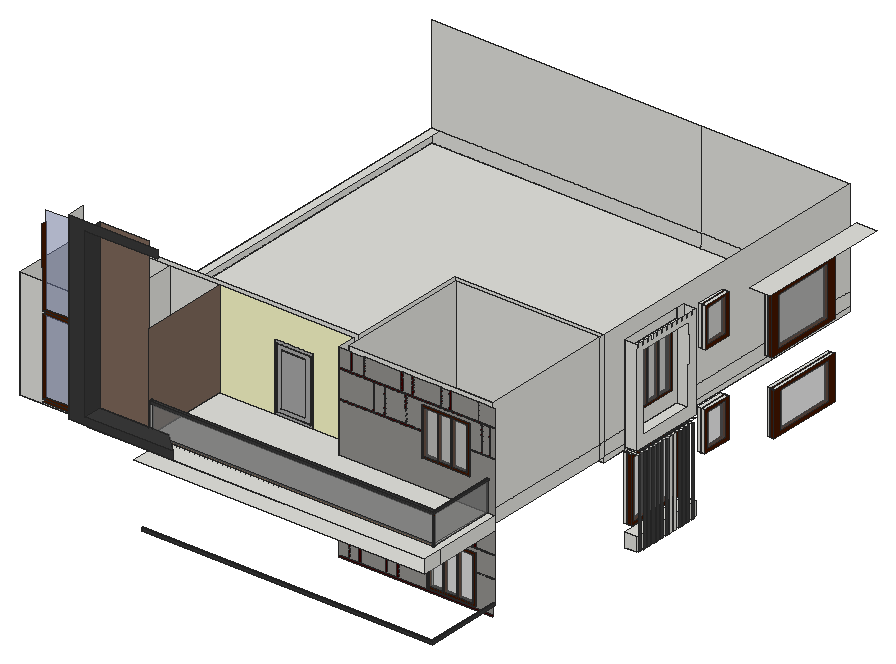
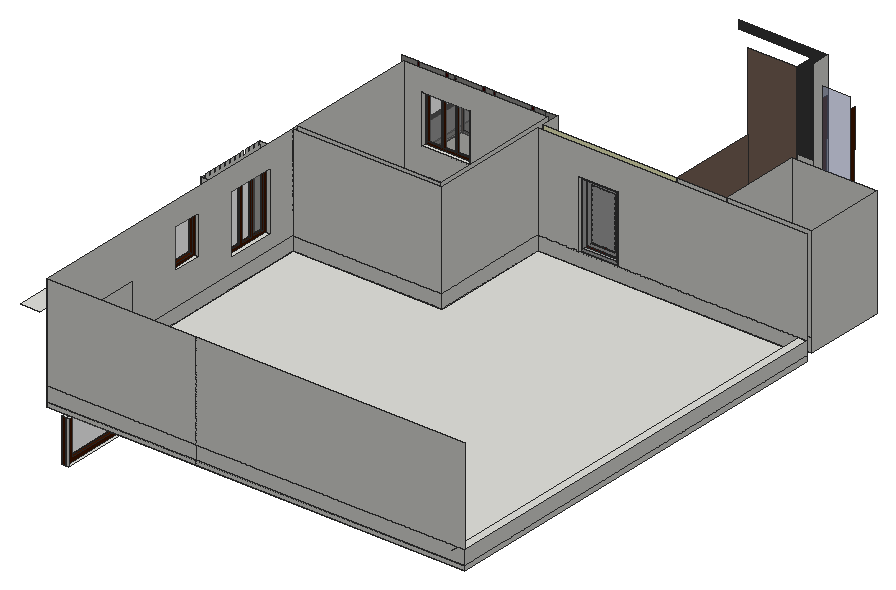
# SketchUp Ruby script. Lengths in inches.
U = 1.inch
M = Sketchup.active_model
def pt(a) = Geom::Point3d.new(a.map { |v| v * U })
def face(e, loops, mat)
  f = e.add_face(loops[0].map { |a| pt(a) })
  loops[1..].each { |l| e.add_face(l.map { |a| pt(a) }).erase! }
  f.material = f.back_material = mat if mat
  f
end
# faces: each face lists its corners as indices into pts; further lists are holes
def faces(e, pts, list, mat = nil) = list.each { |f| face(e, (f[0].is_a?(Array) ? f : [f]).map { |l| l.map { |i| pts[i] } }, mat) }
# xy, xz, yz: faces in a plane at the given z, y or x. An outline is a flat list of corners, or four numbers for a rectangle; further outlines are holes
def ring(l) = l.size == 4 ? [[l[0], l[1]], [l[2], l[1]], [l[2], l[3]], [l[0], l[3]]] : l.each_slice(2).to_a
def flat(e, list, mat, &to3) = list.each { |f| face(e, (f[0].is_a?(Array) ? f : [f]).map { |l| ring(l).map { |u, v| to3.(u, v) } }, mat) }
def xy(e, z, list, mat = nil) = flat(e, list, mat) { |x, y| [x, y, z] }
def xz(e, y, list, mat = nil) = flat(e, list, mat) { |x, z| [x, y, z] }
def yz(e, x, list, mat = nil) = flat(e, list, mat) { |y, z| [x, y, z] }
def lines(e, pts, list) = list.each { |a, b| e.add_line(pt(pts[a]), pt(pts[b])) }
# prism: a flat outline (further loops are holes) pulled along v
def prism(e, loops, v, mat = nil)
  f = face(e, loops, mat); d = Geom::Vector3d.new(v.map { |x| x * U })
  f.pushpull(f.normal.samedirection?(d) ? d.length : -d.length)
end
def box(e, o, s, mat = nil) = prism(e, [[o, [o[0] + s[0], o[1], o[2]], [o[0] + s[0], o[1] + s[1], o[2]], [o[0], o[1] + s[1], o[2]]]], [0, 0, s[2]], mat)
def at(x, y, z, deg = 0) = Geom::Transformation.translation(pt([x, y, z])) * Geom::Transformation.rotation(ORIGIN, Z_AXIS, deg.degrees)
def axes(o, x, y, z) = Geom::Transformation.new([*x, 0, *y, 0, *z, 0, *pt(o).to_a, 1])
def part(name) = M.definitions.add(name)
# library, detail: a bought-in or finely detailed component or shape, given as its bounding box
def library(name, o, s) = part(name).tap { |d| box(d.entities, o, s) }
def detail(e, o, s) = box(e.add_group.entities, o, s)
def put(e, d, t, mat = nil) = e.add_instance(d, t).tap { |i| i.material = mat if mat }
def group(e, t, mat = nil) = e.add_group.tap { |g| g.transformation = t; g.material = mat if mat }.entities
root = M.entities
M.materials.add("[Color A08]").color = [67, 22, 0]
M.materials.add("[Color A08]1").color = [91, 11, 0]
M.materials.add("[Color A08]2").color = [65, 0, 0]
M.materials.add("[Color A08]3").color = [60, 0, 0]
M.materials.add("[Color B08]").color = [69, 25, 0]
M.materials.add("[Color E01]").color = [255, 255, 204]
M.materials.add("[Color M03]").color = [170, 170, 170]
M.materials.add("[Color M07]").color = [58, 58, 58]
M.materials.add("[Granite Brown]").color = [126, 104, 91]
M.materials.add("[Granite Light Gray]").color = [149, 148, 144]
M.materials.add("[Translucent Glass Gray]").color = [128, 128, 128]
M.materials["[Translucent Glass Gray]"].alpha = 0.5
M.materials.add("[Translucent Glass Sky Reflection]").color = [126, 138, 183]
M.materials["[Translucent Glass Sky Reflection]"].alpha = 0.52
M.materials.add("[Wood Floor]").color = [155, 105, 61]
c1 = part("Group\#2")
xy(c1.entities,0,[[0,0,74.4375,5]],"[Color A08]")
xy(c1.entities,4.02,[[4.02,0,24.3,5],[27.19,0,45.86,5],[48.76,0,70.42,5]],"[Color A08]")
xy(c1.entities,85.67,[[4.02,0,24.3,5],[27.19,0,45.86,5],[48.76,0,70.42,5]],"[Color A08]")
xy(c1.entities,89.6875,[[0,0,74.4375,5]],"[Color A08]")
xz(c1.entities,0,[[[0,0,74.4375,89.6875],[48.76,4.02,70.42,85.67],[4.02,4.02,24.3,85.67],[27.19,4.02,45.86,85.67]]],"[Color A08]")
xz(c1.entities,0,[[4.02,4.02,24.3,85.67],[27.19,4.02,45.86,85.67],[48.76,4.02,70.42,85.67]],"[Translucent Glass Gray]")
xz(c1.entities,5,[[[0,0,74.4375,89.6875],[48.76,4.02,70.42,85.67],[4.02,4.02,24.3,85.67],[27.19,4.02,45.86,85.67]]],"[Color A08]")
yz(c1.entities,0,[[0,0,5,89.6875]],"[Color A08]")
yz(c1.entities,4.02,[[0,4.02,5,85.67]],"[Color A08]")
yz(c1.entities,24.3,[[0,4.02,5,85.67]],"[Color A08]")
yz(c1.entities,27.19,[[0,4.02,5,85.67]],"[Color A08]")
yz(c1.entities,45.86,[[0,4.02,5,85.67]],"[Color A08]")
yz(c1.entities,48.76,[[0,4.02,5,85.67]],"[Color A08]")
yz(c1.entities,70.42,[[0,4.02,5,85.67]],"[Color A08]")
yz(c1.entities,74.4375,[[0,0,5,89.6875]],"[Color A08]")
c2 = part("Group\#1")
xy(c2.entities,0,[[0,0,26.5,5]],"[Color A08]")
xy(c2.entities,2.85,[[2.85,0,23.65,5]],"[Color A08]")
xy(c2.entities,35.15,[[2.85,0,23.65,5]],"[Color A08]")
xy(c2.entities,38,[[0,0,26.5,5]],"[Color A08]")
xz(c2.entities,0,[[[0,0,26.5,38],[2.85,2.85,23.65,35.15]]],"[Color A08]")
xz(c2.entities,0,[[2.85,2.85,23.65,35.15]],"[Translucent Glass Gray]")
xz(c2.entities,5,[[[0,0,26.5,38],[2.85,2.85,23.65,35.15]]],"[Color A08]")
yz(c2.entities,0,[[0,0,5,38]],"[Color A08]")
yz(c2.entities,2.85,[[0,2.85,5,35.15]],"[Color A08]")
yz(c2.entities,23.65,[[0,2.85,5,35.15]],"[Color A08]")
yz(c2.entities,26.5,[[0,0,5,38]],"[Color A08]")
c3 = part("Group\#3")
xy(c3.entities,0,[[0,0,48,5]],"[Color M03]")
xy(c3.entities,2.98,[[2.98,0,45.02,5]],"[Color M03]")
xy(c3.entities,81.02,[[2.98,0,45.02,5]],"[Color M03]")
xy(c3.entities,84,[[0,0,48,5]],"[Color M03]")
xz(c3.entities,0,[[[2.98,2.98,45.02,81.02],[4.42,4.42,43.58,79.58]],[[8.55,8.55,39.45,75.45],[9.61,9.61,38.39,74.39]]],"[Color A08]1")
xz(c3.entities,0,[[[0,0,48,84],[2.98,2.98,45.02,81.02]],[[4.42,4.42,43.58,79.58],[8.55,8.55,39.45,75.45]],[9.61,9.61,38.39,74.39]],"[Color M03]")
xz(c3.entities,5,[[[0,0,48,84],[2.98,2.98,45.02,81.02]]],"[Color M03]")
yz(c3.entities,0,[[0,0,5,84]],"[Color M03]")
yz(c3.entities,2.98,[[0,2.98,5,81.02]],"[Color M03]")
yz(c3.entities,45.02,[[0,2.98,5,81.02]],"[Color M03]")
yz(c3.entities,48,[[0,0,5,84]],"[Color M03]")
xy(root,287.863,[[540,318.915,555.511,322.29],[540,325.727,555.511,329.102],[540,332.54,555.511,335.915],[540,339.352,555.511,342.727],[540,346.165,555.511,349.54],
  [540,352.977,555.511,356.352],[540,359.79,555.511,363.165],[540,366.602,555.511,369.977],[540,373.415,555.511,376.79],[540,380.227,555.511,383.602],
  [540,387.04,555.511,390.415],[540,393.852,555.511,397.227],[540.073,400.665,555.511,404.04]])
xy(root,288.911,[[540,316.711,554.5,407.898]])
xy(root,303.188,[[456.001,113.4375,516.001,121.0625]])
xy(root,305.974,[[540,316.711,554.5,407.898]])
xy(root,308.49,[[531,550.287,540,644.037]])
xy(root,308.5625,[[531,326.103,540,399.728]])
xy(root,312.5625,[[176.764,15.4375,176.764,17.368,537.487,17.368,537.487,113.4375,540,113.4375,540,15.4375]])
xy(root,315.5625,[[176.764,15.4375,540,15.4375,540,113.4375,537.487,113.4375,537.487,17.368,176.764,17.368]],"[Color M07]")
xy(root,338.694,[[531,441.389,540,477.826]])
xy(root,360.5625,[[245.49,137.125,293.49,144.4375]])
xy(root,362.365,[[531,550.287,540,644.037]])
xy(root,363.188,[[456.001,113.4375,516.001,121.0625]])
xy(root,387.944,[[531,441.389,540,477.826]])
xy(root,388.5,[[531,326.103,540,399.728]])
xy(root,390.5625,[[9,144.4375,9,678,531,678,531,294,345.1875,294,345.1875,144.4375]])
xy(root,395.819,[[540,318.915,555.511,322.29],[540,325.727,555.511,329.102],[540,332.54,555.511,335.915],[540,339.352,555.511,342.727],[540,346.165,555.511,349.54],
  [540,352.977,555.511,356.352],[540,359.79,555.511,363.165],[540,366.602,555.511,369.977],[540,373.415,555.511,376.79],[540,380.227,555.511,383.602],
  [540,387.04,555.511,390.415],[540,393.852,555.511,397.227],[540,400.665,555.511,404.04]])
xy(root,396.5625,[[176.764,3.875,540,27],[176.656,27,176.764,36],[114.932,36,176.656,137.125],[176.656,36,176.764,137.125],[9,144.4375,345.1875,144.4375,345.1875,294,531,294,531,678,9,678]])
xy(root,396.5625,[[9,36,114.932,137.125]],"[Color E01]")
xy(root,396.5625,[[176.764,27,176.764,137.125,345.1875,137.125,345.1875,113.4375,540,113.4375,540,27]],"[Wood Floor]")
xy(root,400.902,[[531,545.634,540,643.134]])
xy(root,401.881,[[540,316.142,554.5,318.915],[540,318.915,554.5,322.29],[540,322.29,554.5,325.727],[540,325.727,554.5,329.102],[540,329.102,554.5,332.54],
  [540,332.54,554.5,335.915],[540,335.915,554.5,339.352],[540,339.352,554.5,342.727],[540,342.727,554.5,346.165],[540,346.165,554.5,349.54],
  [540,349.54,554.5,352.977],[540,352.977,554.5,356.352],[540,356.352,554.5,359.79],[540,359.79,554.5,363.165],[540,363.165,554.5,366.602],
  [540,366.602,554.5,369.977],[540,369.977,554.5,373.415],[540,373.415,554.5,376.79],[540,376.79,554.5,380.227],[540,380.227,554.5,383.602],
  [540,383.602,554.5,387.04],[540,387.04,554.5,390.415],[540,390.415,554.5,393.852],[540,393.852,554.5,397.227],[540,397.227,554.5,400.665],
  [540,400.665,554.5,404.04],[540,404.04,554.5,408.01]])
xy(root,401.881,[[554.5,318.915,558.125,322.29],[554.5,325.727,558.125,329.102],[554.5,332.54,558.125,335.915],[554.5,339.352,558.125,342.727],[554.5,346.165,558.125,349.54],
  [554.5,352.977,558.125,356.352],[554.5,359.79,558.125,363.165],[554.5,366.602,558.125,369.977],[554.5,373.415,558.125,376.79],[554.5,380.227,558.125,383.602],
  [554.5,387.04,558.125,390.415],[554.5,393.852,558.125,397.227],[554.5,400.665,558.125,404.04]],"[Color M07]")
xy(root,408.171,[[47.934,22.1875,82.843,27]],"[Color B08]")
xy(root,411.105,[[47.944,22.1875,82.854,27]],"[Color B08]")
xy(root,413.5625,[[94.799,3.875,114.932,27],[114.932,3.875,122.065,27],[122.065,3.875,122.065,27,201.085,27,224.863,3.875],[224.863,3.875,540,3.875,540,113.4375,532.387,113.4375,532.387,27,201.085,27],[176.656,27,176.764,137.125],
  [176.764,31.5,529.965,31.5,529.965,113.4375,345.1875,113.4375,345.1875,137.125,293.49,137.125,293.49,144.4375,245.49,144.4375,245.49,137.125,176.764,137.125],[351.1875,121.0625,531,288],[9,144.4375,18.8125,678]])
xy(root,415.784,[[540,325.42,554.5,396.295]])
xy(root,423.1875,[[114.932,3.875,224.863,3.875,201.085,27,114.932,27]],"[Color M07]")
xy(root,431.081,[[531,329.523,540,390.773]])
xy(root,446.074,[[448.284,113.4375,508.284,121.0625]])
xy(root,449.5625,[[176.764,27,178.309,31.5],[178.309,27,178.309,31.5,529.965,31.5,529.965,113.4375,532.387,113.4375,532.387,27]])
xy(root,452.5625,[[176.764,27,178.309,31.5],[178.309,27,532.387,27,532.387,113.4375,529.965,113.4375,529.965,31.5,178.309,31.5]],"[Color M07]")
xy(root,455.034,[[531,441.79,540,478.227]])
xy(root,472.214,[[531,545.634,540,643.134]])
xy(root,493.645,[[540,510.973,564.9375,677.392]])
xy(root,497.5625,[[245.49,137.125,293.49,144.4375]])
xy(root,504.284,[[531,441.79,540,478.227]])
xy(root,505.331,[[531,329.523,540,390.773]])
xy(root,506.074,[[448.284,113.4375,508.284,121.0625]])
xy(root,506.734,[[48.291,22.1875,83.2,27]],"[Color B08]")
xy(root,509.668,[[48.291,22.1875,83.2,27]],"[Color B08]")
xy(root,510.846,[[540,325.42,554.5,397.041]])
xz(root,3.875,[[94.799,413.5625,224.863,413.5625,224.863,423.1875,114.932,423.1875,114.932,631.3125,205.994,631.3125,205.994,641.625,94.799,641.625]],"[Color M07]")
xz(root,15.4375,[[176.764,312.5625,540,315.5625]],"[Color M07]")
xz(root,17.368,[[176.764,312.5625,537.487,315.5625]],"[Color M07]")
xz(root,27,[[114.932,396.5625,122.065,413.5625],[176.764,396.5625,345.1875,413.5625],[94.799,413.5625,176.656,413.5625,176.656,423.1875,114.932,423.1875,114.932,533.5625,94.799,533.5625],[176.656,413.5625,176.764,423.1875],[176.764,413.5625,178.309,423.1875],
  [178.309,413.5625,201.085,423.1875],[531.09,449.5625,532.387,452.5625]])
xz(root,27,[[531.09,413.5625,532.387,449.5625]],"[Color A08]")
xz(root,27,[[176.764,423.1875,178.309,449.5625],[176.764,449.5625,178.309,452.5625],[178.309,449.5625,531.09,452.5625]],"[Color M07]")
xz(root,27,[[114.932,423.1875,176.764,631.3125]],"[Granite Brown]")
xz(root,27,[[201.085,413.5625,531.09,413.5625,531.09,449.5625,178.309,449.5625,178.309,423.1875,201.085,423.1875]],"[Translucent Glass Gray]")
xz(root,27,[[47.944,411.105,82.854,411.105,83.2,506.734,48.291,506.734],[48.291,509.668,83.2,509.668,82.402,607.668,82.402,621.293,47.493,621.293,47.493,607.668]],"[Translucent Glass Sky Reflection]")
xz(root,31.5,[[176.764,413.5625,178.309,449.5625],[176.764,449.5625,178.309,452.5625],[178.309,449.5625,529.965,452.5625]],"[Color M07]")
xz(root,31.5,[[178.309,413.5625,528.377,449.5625],[528.377,413.5625,529.965,449.5625]],"[Translucent Glass Gray]")
xz(root,36,[[9,396.5625,114.932,533.5625]])
xz(root,113.4375,[[537.487,312.5625,540,315.5625],[529.965,449.5625,532.387,452.5625]])
xz(root,113.4375,[[345.1875,475.328,448.284,475.638,448.284,477.542,389.772,477.542,387.762,477.536,387.762,477.542,345.1875,477.542],[508.284,475.818,540,475.914,540,477.542,508.284,477.542],[387.762,477.542,389.772,477.542,389.675,509.774,387.665,509.768],[401.325,477.542,403.335,477.542,403.238,509.774,401.228,509.768],[427.887,477.542,429.897,477.542,429.8,509.774,427.79,509.768],
  [435.512,477.542,437.522,477.542,437.425,509.774,435.415,509.768],[522.262,477.542,524.272,477.542,524.175,509.774,522.165,509.768],[532.45,477.542,534.46,477.542,534.363,509.774,532.353,509.768],[345.1875,509.64,387.665,509.768,389.675,509.774,540,510.226,540,511.855,345.1875,511.855],[359.208,511.855,361.427,533.5625],
  [374.645,511.855,376.865,533.5625],[422.208,511.855,424.427,533.5625],[436.145,511.855,438.365,533.5625],[471.77,511.855,473.99,533.5625],[482.77,511.855,484.99,533.5625],
  [517.833,511.855,520.052,533.5625]],"[Color A08]2")
xz(root,113.4375,[[345.1875,299.249,537.487,301.895],[357.064,301.895,359.076,340.135],[369.752,301.895,371.764,340.135],[403.064,301.895,405.076,340.135],[417.689,301.895,419.701,340.135],
  [345.1875,340.135,455.324,341.815],[516.796,341.526,540,342.887],[382.892,341.815,385.032,368.215],[392.079,341.815,394.22,368.215],[429.454,341.815,431.595,368.215],
  [437.017,341.815,439.157,368.215],[345.1875,368.215,540,370.151],[360.348,370.151,362.091,396.5625],[371.536,370.151,373.279,396.5625],[406.973,370.151,408.716,396.5625],
  [419.661,370.151,421.404,396.5625],[447.161,370.151,448.904,396.5625],[459.161,370.151,460.904,396.5625],[504.536,370.151,506.279,396.5625],[513.973,370.151,515.716,396.5625]],"[Color A08]3")
xz(root,113.4375,[[345.1875,301.895,357.064,340.135],[359.076,301.895,369.752,340.135],[371.764,301.895,403.064,340.135],[405.076,301.895,417.689,340.135],[[419.701,301.895,537.487,301.895,537.487,315.5625,540,315.5625,540,341.526,516.796,341.526,516.796,342.887,540,342.887,540,368.215,439.157,368.215,439.157,341.815,455.324,341.815,455.324,340.135,419.701,340.135],[456.001,303.188,516.001,363.188]],
  [345.1875,341.815,382.892,368.215],[385.032,341.815,392.079,368.215],[394.22,341.815,429.454,368.215],[431.595,341.815,437.017,368.215],[345.1875,370.151,360.348,396.5625],
  [362.091,370.151,371.536,396.5625],[373.279,370.151,406.973,396.5625],[408.716,370.151,419.661,396.5625],[421.404,370.151,447.161,396.5625],[448.904,370.151,459.161,396.5625],
  [460.904,370.151,504.536,396.5625],[506.279,370.151,513.973,396.5625],[515.716,370.151,540,396.5625],[345.1875,413.5625,529.965,413.5625,529.965,452.5625,532.387,452.5625,532.387,413.5625,540,413.5625,540,475.914,508.284,475.818,508.284,446.074,448.284,446.074,448.284,475.638,345.1875,475.328],[387.762,477.536,389.772,477.542,387.762,477.542],
  [345.1875,477.542,387.762,477.542,387.665,509.768,345.1875,509.64],[389.772,477.542,401.325,477.542,401.228,509.768,403.238,509.774,403.335,477.542,427.887,477.542,427.79,509.768,429.8,509.774,429.897,477.542,435.512,477.542,435.415,509.768,437.425,509.774,437.522,477.542,448.284,477.542,448.284,506.074,508.284,506.074,508.284,477.542,522.262,477.542,522.165,509.768,524.175,509.774,524.272,477.542,532.45,477.542,532.353,509.768,534.363,509.774,534.46,477.542,540,477.542,540,510.226,389.675,509.774],[345.1875,511.855,359.208,533.5625],[361.427,511.855,374.645,533.5625],[376.865,511.855,422.208,533.5625],
  [424.427,511.855,436.145,533.5625],[438.365,511.855,471.77,533.5625],[473.99,511.855,482.77,533.5625],[484.99,511.855,517.833,533.5625],[520.052,511.855,540,533.5625]],"[Granite Light Gray]")
xz(root,121.0625,[[351.1875,396.5625,531,413.5625],[[351.1875,413.5625,531,533.5625],[448.284,446.074,508.284,506.074]]])
xz(root,137.125,[[9,396.5625,114.932,413.5625],[114.932,396.5625,176.656,413.5625],[176.656,396.5625,176.764,413.5625],[9,413.5625,114.932,533.5625],[114.932,413.5625,176.764,533.5625]])
xz(root,137.125,[[176.764,413.5625,245.49,413.5625,245.49,497.5625,293.49,497.5625,293.49,413.5625,345.1875,413.5625,345.1875,533.5625,176.764,533.5625]],"[Color E01]")
xz(root,144.4375,[[9,390.5625,345.1875,396.5625],[9,396.5625,345.1875,413.5625],[9,413.5625,9,533.5625,345.1875,533.5625,345.1875,413.5625,293.49,413.5625,293.49,497.5625,245.49,497.5625,245.49,413.5625]])
xz(root,288,[[351.1875,396.5625,531,413.5625],[351.1875,413.5625,531,533.5625]])
xz(root,294,[[345.1875,390.5625,531,396.5625],[345.1875,396.5625,531,413.5625],[345.1875,413.5625,531,533.5625]])
xz(root,316.142,[[540,401.881,554.5,521.096]])
xz(root,316.711,[[540,288.911,554.5,305.974]])
xz(root,325.42,[[540,415.784,554.5,510.846]])
xz(root,326.103,[[531,308.5625,540,388.5]])
xz(root,329.523,[[531,431.081,540,505.331]])
xz(root,390.773,[[531,431.081,540,505.331]])
xz(root,399.728,[[531,308.5625,540,388.5]])
xz(root,407.898,[[540,288.911,554.5,305.974]])
xz(root,408.01,[[540,401.881,554.5,521.096]])
xz(root,441.389,[[531,338.694,540,387.944]])
xz(root,441.79,[[531,455.034,540,504.284]])
xz(root,477.826,[[531,338.694,540,387.944]])
xz(root,478.227,[[531,455.034,540,504.284]])
xz(root,545.634,[[531,400.902,540,472.214]])
xz(root,550.287,[[531,308.49,540,362.365]])
xz(root,643.134,[[531,400.902,540,472.214]])
xz(root,644.037,[[531,308.49,540,362.365]])
xz(root,678,[[9,390.5625,345.75,396.5625],[345.75,390.5625,531,396.5625],[9,396.5625,345.75,413.5625],[345.75,396.5625,531,413.5625],[9,413.5625,345.75,533.5625],
  [345.75,413.5625,531,533.5625]])
yz(root,9,[[144.4375,390.5625,678,396.5625],[36,396.5625,137.125,533.5625],[144.4375,396.5625,678,413.5625]])
yz(root,94.799,[[3.875,413.5625,27,641.625]])
yz(root,114.932,[[36,396.5625,137.125,533.5625]])
yz(root,114.932,[[3.875,423.1875,27,631.3125]],"[Color M07]")
yz(root,176.656,[[27,396.5625,137.125,413.5625]])
yz(root,176.764,[[15.4375,312.5625,17.368,315.5625],[27,396.5625,137.125,413.5625],[27,413.5625,31.5,449.5625],[27,449.5625,31.5,452.5625]])
yz(root,176.764,[[31.5,413.5625,137.125,413.5625,137.125,533.5625,27,533.5625,27,452.5625,31.5,452.5625]],"[Granite Brown]")
yz(root,178.309,[[27,449.5625,31.5,452.5625]])
yz(root,245.49,[[137.125,413.5625,144.4375,497.5625]])
yz(root,293.49,[[137.125,413.5625,144.4375,497.5625]])
yz(root,345.1875,[[144.4375,390.5625,294,396.5625],[144.4375,396.5625,294,413.5625],[113.4375,413.5625,137.125,533.5625],[144.4375,413.5625,294,533.5625]])
yz(root,351.1875,[[121.0625,396.5625,288,413.5625],[121.0625,413.5625,288,533.5625]])
yz(root,448.284,[[113.4375,446.074,121.0625,506.074]])
yz(root,456.001,[[113.4375,303.188,121.0625,363.188]])
yz(root,508.284,[[113.4375,446.074,121.0625,506.074]])
yz(root,516.001,[[113.4375,303.188,121.0625,363.188]])
yz(root,529.965,[[31.5,449.5625,113.4375,452.5625]],"[Color M07]")
yz(root,529.965,[[31.5,413.5625,32.527,449.5625],[32.527,413.5625,113.4375,449.5625]],"[Translucent Glass Gray]")
yz(root,531,[[326.103,388.5,399.728,390.5625],[294,390.5625,326.103,396.5625],[326.103,390.5625,399.728,396.5625],[399.728,390.5625,678,396.5625],[121.0625,396.5625,288,413.5625],
  [288,396.5625,294,413.5625],[294,396.5625,294,413.5625,545.634,413.5625,545.634,400.902,643.134,400.902,643.134,413.5625,678,413.5625,678,396.5625],[545.634,400.902,643.134,472.214],[121.0625,413.5625,288,533.5625],[288,413.5625,294,533.5625],
  [[294,413.5625,294,533.5625,678,533.5625,678,413.5625,643.134,413.5625,643.134,472.214,545.634,472.214,545.634,413.5625],[329.523,431.081,390.773,505.331],[441.79,455.034,478.227,504.284]]])
yz(root,532.387,[[27,413.5625,29.298,449.5625]],"[Color A08]")
yz(root,532.387,[[27,449.5625,29.298,452.5625],[29.298,449.5625,113.4375,452.5625]],"[Color M07]")
yz(root,532.387,[[29.298,413.5625,113.4375,449.5625]],"[Translucent Glass Gray]")
yz(root,537.487,[[17.368,312.5625,113.4375,315.5625]],"[Color M07]")
yz(root,540,[[339.352,395.819,342.727,401.881],[346.165,395.819,349.54,401.881],[352.977,395.819,356.352,401.881],[359.79,395.819,363.165,401.881],[366.602,395.819,369.977,401.881],
  [373.415,395.819,376.79,401.881],[380.227,395.819,383.602,401.881],[387.04,395.819,390.415,401.881],[393.852,395.819,397.227,401.881],[400.665,395.819,404.04,401.881],
  [3.875,396.5625,27,413.5625],[27,396.5625,113.4375,413.5625],[316.142,401.881,316.142,521.096,397.041,521.096,397.041,510.846,325.42,510.846,325.42,415.784,396.295,415.784,396.373,415.783,397.041,510.846,397.12,521.096,408.01,521.096,408.01,401.881],[[396.373,415.783,397.041,510.846,397.12,521.096,397.041,521.096,397.041,510.846,325.42,510.846,325.42,415.784,396.295,415.784],[329.523,431.081,390.773,505.331]]])
yz(root,540,[[15.4375,312.5625,113.4375,315.5625]],"[Color M07]")
yz(root,554.5,[[316.711,288.911,407.898,305.974],[[316.142,401.881,408.01,401.881,408.01,521.096,404.267,521.096,404.267,516.096,400.892,516.096,400.892,521.096,395.767,521.096,395.767,516.096,392.392,516.096,392.392,521.096,388.142,521.096,388.142,516.096,384.767,516.096,384.767,521.096,380.517,521.096,380.517,516.096,377.142,516.096,377.142,521.096,372.892,521.096,372.892,516.096,369.517,516.096,369.517,521.096,365.267,521.096,365.267,516.096,361.892,516.096,361.892,521.096,357.642,521.096,357.642,516.096,354.267,516.096,354.267,521.096,350.017,521.096,350.017,516.096,346.642,516.096,346.642,521.096,342.392,521.096,342.392,516.096,339.017,516.096,339.017,521.096,334.767,521.096,334.767,516.096,331.392,516.096,331.392,521.096,327.142,521.096,327.142,516.096,323.767,516.096,323.767,521.096,319.517,521.096,319.517,516.096,316.142,516.096],[396.373,415.783,396.295,415.784,325.42,415.784,325.42,510.846,397.041,510.846]]])
yz(root,555.511,[[366.602,287.863,369.977,395.819],[373.415,287.863,376.79,395.819]])
yz(root,555.511,[[318.915,287.863,322.29,395.819],[325.727,287.863,329.102,395.819],[332.54,287.863,335.915,395.819],[339.352,287.863,342.727,395.819],[346.165,287.863,349.54,395.819],
  [352.977,287.863,356.352,395.819],[359.79,287.863,363.165,395.819],[380.227,287.863,383.602,395.819],[387.04,287.863,390.415,395.819],[393.852,287.863,397.227,395.819],
  [400.665,287.863,404.04,395.819]],"[Color M07]")
p = [[47.944,27,411.105],[48.291,27,506.734],[48.291,22.1875,506.734],[47.944,22.1875,411.105],[83.2,27,506.734],[82.854,27,411.105],
  [82.854,22.1875,411.105],[83.2,22.1875,506.734],[224.863,3.875,413.5625],[201.085,27,413.5625],[201.085,27,423.1875],[224.863,3.875,423.1875],
  [540,396.295,415.784],[554.5,396.295,415.784],[554.5,396.373,415.783],[540,396.373,415.783],[554.5,397.041,510.846],[540,397.041,510.846],
  [48.291,27,509.668],[47.493,27,607.668],[47.493,22.1875,607.668],[48.291,22.1875,509.668],[82.402,27,607.668],[83.2,27,509.668],
  [83.2,22.1875,509.668],[82.402,22.1875,607.668],[18.8125,137.125,413.5625],[18.8125,144.4375,413.5625],[18.8125,678,413.5625],[18.8125,687,413.5625]]
faces(root,p,[[0,1,2,3],[4,5,6,7],[18,19,20,21],[22,23,24,25]],"[Color B08]")
faces(root,p,[[8,9,10,11],[12,13,14,15],[14,16,17,15]])
lines(root,p,[[26,27],[28,29]])
put(root,c1,axes([455.32,113.4375,303.1875],[0.81514,0,0],[0,0.39878,0],[0,0,0.66899]))
put(root,c2,axes([540,548.92,308.49],[0,3.58944,0],[-1,0,0],[0,0,1.41776]))
put(root,c1,axes([540,326.1,308.5625],[0,0.98912,0],[-1.23966,0,0],[0,0,0.89013]),"[Color M07]")
put(root,c2,axes([540,441.39,338.69],[0,1.375,0],[-1,0,0],[0,0,1.29605]))
put(root,c2,axes([540,545.63,400.9],[0,3.67925,0],[-1,0,0],[0,0,1.87664]))
put(root,c3,at(245.49,137.125,413.5625))
put(root,c1,axes([540,329.52,431.08],[0,0.82284,0],[-0.66942,0,0],[0,0,0.82787]))
put(root,c1,axes([448.21,113.46,446.07],[0.80699,0,0],[0,0.3948,0],[0,0,0.66899]))
put(root,c2,axes([540,441.79,455.03],[0,1.375,0],[-1,0,0],[0,0,1.29605]))
